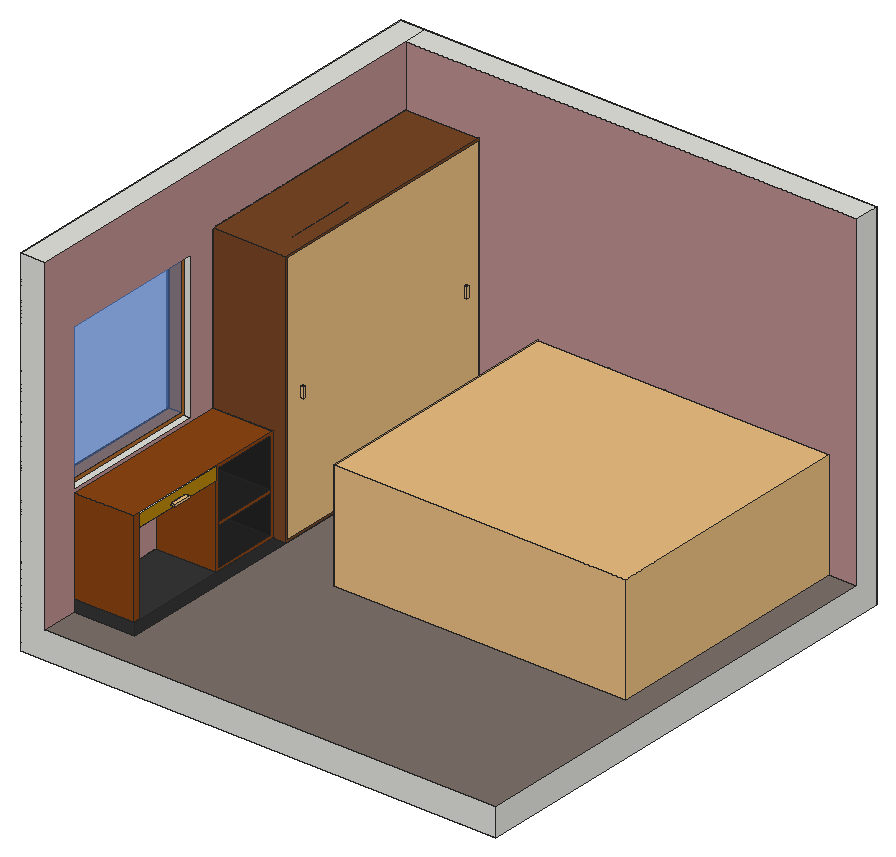
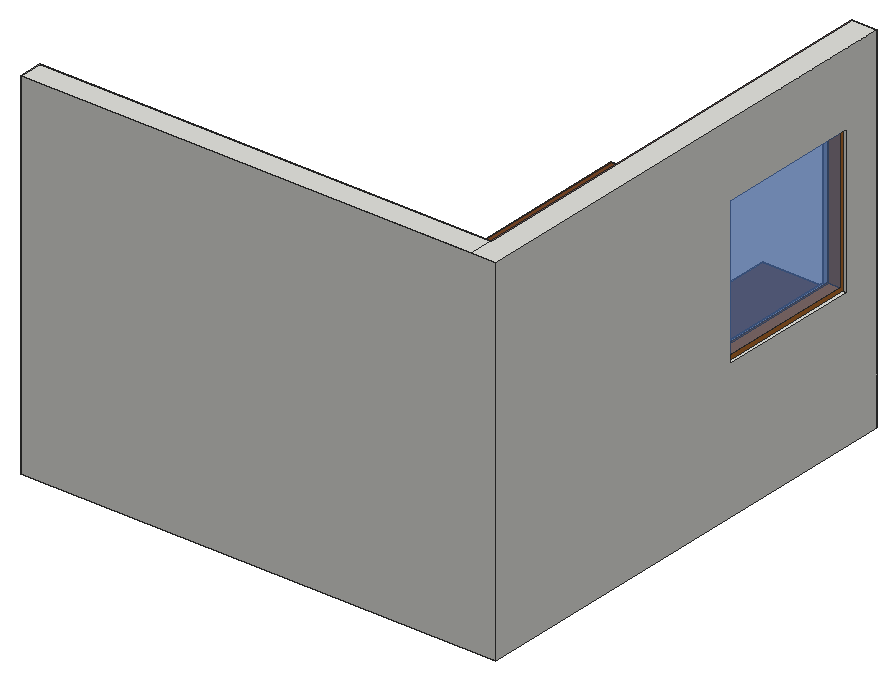
# SketchUp Ruby script. Lengths in inches.
U = 1.inch
M = Sketchup.active_model
def pt(a) = Geom::Point3d.new(a.map { |v| v * U })
def face(e, loops, mat)
  f = e.add_face(loops[0].map { |a| pt(a) })
  loops[1..].each { |l| e.add_face(l.map { |a| pt(a) }).erase! }
  f.material = f.back_material = mat if mat
  f
end
# faces: each face lists its corners as indices into pts; further lists are holes
def faces(e, pts, list, mat = nil) = list.each { |f| face(e, (f[0].is_a?(Array) ? f : [f]).map { |l| l.map { |i| pts[i] } }, mat) }
# xy, xz, yz: faces in a plane at the given z, y or x. An outline is a flat list of corners, or four numbers for a rectangle; further outlines are holes
def ring(l) = l.size == 4 ? [[l[0], l[1]], [l[2], l[1]], [l[2], l[3]], [l[0], l[3]]] : l.each_slice(2).to_a
def flat(e, list, mat, &to3) = list.each { |f| face(e, (f[0].is_a?(Array) ? f : [f]).map { |l| ring(l).map { |u, v| to3.(u, v) } }, mat) }
def xy(e, z, list, mat = nil) = flat(e, list, mat) { |x, y| [x, y, z] }
def xz(e, y, list, mat = nil) = flat(e, list, mat) { |x, z| [x, y, z] }
def yz(e, x, list, mat = nil) = flat(e, list, mat) { |y, z| [x, y, z] }
def lines(e, pts, list) = list.each { |a, b| e.add_line(pt(pts[a]), pt(pts[b])) }
# prism: a flat outline (further loops are holes) pulled along v
def prism(e, loops, v, mat = nil)
  f = face(e, loops, mat); d = Geom::Vector3d.new(v.map { |x| x * U })
  f.pushpull(f.normal.samedirection?(d) ? d.length : -d.length)
end
def box(e, o, s, mat = nil) = prism(e, [[o, [o[0] + s[0], o[1], o[2]], [o[0] + s[0], o[1] + s[1], o[2]], [o[0], o[1] + s[1], o[2]]]], [0, 0, s[2]], mat)
def at(x, y, z, deg = 0) = Geom::Transformation.translation(pt([x, y, z])) * Geom::Transformation.rotation(ORIGIN, Z_AXIS, deg.degrees)
def axes(o, x, y, z) = Geom::Transformation.new([*x, 0, *y, 0, *z, 0, *pt(o).to_a, 1])
def part(name) = M.definitions.add(name)
# library, detail: a bought-in or finely detailed component or shape, given as its bounding box
def library(name, o, s) = part(name).tap { |d| box(d.entities, o, s) }
def detail(e, o, s) = box(e.add_group.entities, o, s)
def put(e, d, t, mat = nil) = e.add_instance(d, t).tap { |i| i.material = mat if mat }
def group(e, t, mat = nil) = e.add_group.tap { |g| g.transformation = t; g.material = mat if mat }.entities
root = M.entities
M.materials.add("[0043_SaddleBrown]").color = [139, 69, 19]
M.materials.add("[0044_DarkGoldenrod]").color = [184, 134, 11]
M.materials.add("[0119_RosyBrown]").color = [188, 143, 143]
M.materials.add("[0136_Charcoal]").color = [35, 35, 35]
M.materials.add("[Color E01]").color = [255, 255, 204]
M.materials.add("[Color M00]").color = [255, 255, 255]
M.materials.add("[Slate Light Tile]").color = [54, 54, 54]
M.materials.add("[Tile Checker BW]").color = [125, 112, 107]
M.materials.add("[Translucent_Glass_Blue]").color = [100, 149, 237]
M.materials["[Translucent_Glass_Blue]"].alpha = 0.5
M.materials.add("[Wood Veneer 01]").color = [120, 70, 37]
M.materials.add("[Wood_Bamboo_Medium]").color = [177, 105, 43]
c1 = library("Platform bed",[0,0,0],[83.59,95.6,35.43])
c2 = part("Untitled")
xy(c2.entities,34.68,[[46.57,0,194.75,6.75]])
xy(c2.entities,36.94,[[49.13,0,192.19,6.75]],"[Wood_Bamboo_Medium]")
xy(c2.entities,126.69,[[49.13,0,192.19,6.75]],"[Wood_Bamboo_Medium]")
xy(c2.entities,128.49,[[46.57,0,194.75,6.75]],"[Wood_Bamboo_Medium]")
xz(c2.entities,0,[[49.13,36.94,192.19,126.69]],"[Translucent_Glass_Blue]")
xz(c2.entities,0,[[[46.57,34.68,194.75,128.49],[49.13,36.94,192.19,126.69]]],"[Wood_Bamboo_Medium]")
xz(c2.entities,6.75,[[49.13,36.94,192.19,126.69]],"[Translucent_Glass_Blue]")
xz(c2.entities,6.75,[[[46.57,34.68,194.75,128.49],[49.13,36.94,192.19,126.69]]],"[Wood_Bamboo_Medium]")
yz(c2.entities,46.57,[[0,34.68,6.75,128.49]],"[Wood_Bamboo_Medium]")
yz(c2.entities,49.13,[[0,36.94,6.75,126.69]],"[Wood_Bamboo_Medium]")
yz(c2.entities,192.19,[[0,36.94,6.75,126.69]],"[Wood_Bamboo_Medium]")
yz(c2.entities,194.75,[[0,34.68,6.75,128.49]])
c3 = library("1-POIGNEE CLC2\#1",[-3.03,-0.375,0],[6.06,0.75,1.42])
c4 = library("Group\#2",[128,-0.28,0],[77.78,1.7,82.58])
put(root,c1,at(146.95,64.41,9,90))
put(root,c2,axes([5.625,-3.08,27.26],[0,0.32391,0],[-0.62,0,0],[0,0,0.51166]))
g1 = group(root,at(0,0,0))
xy(g1,0,[[0,0,156,156]])
xy(g1,9,[[8,0,156,148]],"[Tile Checker BW]")
xy(g1,45,[[0,12,8,60]])
xy(g1,93,[[0,12,8,60]])
xy(g1,117,[[0,0,8,156],[8,148,156,156]])
xz(g1,0,[[0,0,156,0,156,9,8,9,8,117,0,117]])
xz(g1,12,[[0,45,8,93]])
xz(g1,60,[[0,45,8,93]])
xz(g1,148,[[8,9,156,117]],"[0119_RosyBrown]")
xz(g1,156,[[0,0,156,117]])
yz(g1,0,[[[0,0,156,117],[12,45,60,93]]])
yz(g1,8,[[[0,9,148,117],[12,45,60,93]]],"[0119_RosyBrown]")
yz(g1,156,[[0,0,156,0,156,117,148,117,148,9,0,9]])
g2 = group(root,at(8,68.01,9))
detail(g2,[24,6.31,44.22],[1.42,0.75,3.58])
detail(g2,[24,73.44,44.22],[1.42,0.75,3.58])
g3 = group(g2,at(24,0.79,0,90))
xy(g3,0,[[-56.8,4,79.2,24]])
xy(g3,4,[[0,4,79.2,24]])
xy(g3,4,[[-56.8,4,-54.8,4.25],[-23.37,4,0,4.25]],"[Color M00]")
xy(g3,4,[[-54.8,4,-23.37,24],[-56.8,4.25,-54.8,24],[-23.37,4.25,0,24]],"[Slate Light Tile]")
xy(g3,4,[[0,0,79.2,4]],"[Wood Veneer 01]")
xy(g3,4.71,[[0.71,0,78.49,0.71],[0.71,0.71,78.49,1.42],[0.71,1.42,39.25,22],[39.95,1.42,78.49,22]])
xy(g3,4.71,[[-22.66,4.25,-0.71,24]],"[0136_Charcoal]")
xy(g3,17.47,[[-22.66,4.25,-0.71,24]],"[0136_Charcoal]")
xy(g3,18.18,[[-22.66,4.25,-0.71,24]],"[0136_Charcoal]")
xy(g3,21.65,[[0.71,1.42,19.62,22],[19.62,1.42,20.33,22],[20.33,1.42,39.25,22],[39.95,1.42,58.87,22],[58.87,1.42,59.58,22],
  [59.58,1.42,78.49,22]])
xy(g3,22.35,[[0.71,1.42,19.62,22],[20.33,1.42,39.25,22],[39.95,1.42,58.87,22],[59.58,1.42,78.49,22]])
xy(g3,30.95,[[-54.8,4.25,-23.37,24]],"[Color M00]")
xy(g3,31.11,[[-54.64,4,-23.52,4.25]],"[Color M00]")
xy(g3,34.49,[[-22.66,4.25,-0.71,24]],"[0136_Charcoal]")
xy(g3,35.04,[[-54.64,4,-23.52,4.25]],"[Color M00]")
xy(g3,35.2,[[-56.8,4.25,0,24]],"[0043_SaddleBrown]")
xy(g3,40,[[0.71,1.42,19.62,22],[20.33,1.42,39.25,22],[39.95,1.42,58.87,22],[59.58,1.42,78.49,22]])
xy(g3,46,[[0.71,1.42,39.25,22],[39.95,1.42,78.49,22]])
xy(g3,59.41,[[39.95,1.42,58.87,22],[58.87,1.42,59.58,22],[59.58,1.42,78.49,22]])
xy(g3,60.12,[[39.95,1.42,58.87,22],[59.58,1.42,78.49,22]])
xy(g3,73.17,[[39.95,1.42,58.87,22],[59.58,1.42,78.49,22]])
xy(g3,73.88,[[39.95,1.42,59.22,22],[59.22,1.42,78.49,22]])
xy(g3,82.29,[[0.71,11.65,39.25,11.71],[0.71,11.71,39.25,11.77]])
xy(g3,84.29,[[0.71,11.65,39.25,11.71],[0.71,11.71,39.25,11.77]])
xy(g3,87.29,[[0.71,0,78.49,0.71],[0.71,0.71,78.49,1.42],[0.71,1.42,39.25,22],[39.95,1.42,78.49,22]])
xy(g3,88,[[0,0,79.2,24]],"[Wood Veneer 01]")
xz(g3,0,[[[0,4,79.2,88],[0.71,4.71,78.49,87.29]]],"[Wood Veneer 01]")
xz(g3,1.42,[[39.25,4.71,39.95,87.29],[0.71,21.65,39.25,21.65,39.25,22.35,20.33,22.35,20.33,40,19.62,40,19.62,22.35,0.71,22.35],[39.95,21.65,78.49,21.65,78.49,22.35,59.58,22.35,59.58,40,58.87,40,58.87,22.35,39.95,22.35],[[0.71,40,39.25,46],[0.83,40.12,19.86,45.88],[20.1,40.12,39.13,45.88]],[[39.95,40,78.49,46],[59.34,40.12,78.375,45.88],[40.07,40.12,59.1,45.88]],
  [0.83,40.12,19.86,45.88],[20.1,40.12,39.13,45.88],[40.07,40.12,59.1,45.88],[59.34,40.12,78.375,45.88],[39.95,59.41,78.49,60.12],
  [58.87,60.12,59.58,73.17],[39.95,73.17,78.49,73.88]])
xz(g3,4,[[-54.64,31.11,-23.52,35.04]],"[0044_DarkGoldenrod]")
xz(g3,4,[[-56.8,0,79.2,4]],"[Slate Light Tile]")
xz(g3,4.25,[[-56.8,4,-54.8,35.2],[[-23.37,4,0,35.2],[-22.66,4.71,-0.71,34.49]],[-22.66,17.47,-0.71,18.18]],"[0043_SaddleBrown]")
xz(g3,4.25,[[[-54.8,30.95,-23.37,35.2],[-54.64,31.11,-23.52,35.04]]],"[Color M00]")
xz(g3,10.71,[[0.71,83.23,39.25,83.29],[0.71,83.29,39.25,83.35]])
xz(g3,12.71,[[0.71,83.23,39.25,83.29],[0.71,83.29,39.25,83.35]])
xz(g3,22,[[0.71,4.71,39.25,21.65],[39.95,4.71,78.49,21.65],[0.71,22.35,19.62,40],[20.33,22.35,39.25,40],[39.95,22.35,58.87,40],
  [59.58,22.35,78.49,40],[0.71,46,39.25,87.29],[39.95,46,78.49,59.41],[39.95,60.12,58.87,73.17],[59.58,60.12,78.49,73.17],
  [39.95,73.88,78.49,87.29]])
xz(g3,24,[[-56.8,0,79.2,4],[0,4,79.2,88]])
xz(g3,24,[[[-56.8,4,-56.8,35.2,0,35.2,0,4,-23.37,4,-23.37,30.95,-54.8,30.95,-54.8,4],[-22.66,18.18,-0.71,34.49],[-22.66,4.71,-0.71,17.47]]],"[Slate Light Tile]")
yz(g3,-56.8,[[4.25,4,24,35.2]],"[0043_SaddleBrown]")
yz(g3,-56.8,[[4,0,24,4]],"[Slate Light Tile]")
yz(g3,-54.8,[[4.25,4,24,30.95]],"[0043_SaddleBrown]")
yz(g3,-54.64,[[4,31.11,4.25,35.04]],"[Color M00]")
yz(g3,-23.52,[[4,31.11,4.25,35.04]],"[Color M00]")
yz(g3,-23.37,[[4.25,4,24,30.95]],"[0043_SaddleBrown]")
yz(g3,-22.66,[[4.25,4.71,24,17.47],[4.25,18.18,24,30.95],[4.25,30.95,24,34.49]],"[0136_Charcoal]")
yz(g3,-0.71,[[4.25,4.71,24,17.47],[4.25,18.18,24,34.49]],"[0136_Charcoal]")
yz(g3,0,[[4.25,4,24,35.2]],"[Slate Light Tile]")
yz(g3,0,[[0,4,0,88,24,88,24,35.2,4.25,35.2,4.25,4]],"[Wood Veneer 01]")
yz(g3,0.71,[[0,4.71,0.71,87.29],[0.71,4.71,1.42,87.29],[1.42,4.71,22,21.65],[1.42,22.35,22,40],[[1.42,46,22,87.29],[11.65,82.29,11.58,82.3,11.46,82.32,11.34,82.36,11.28,82.39,11.23,82.42,11.17,82.45,11.12,82.48,11.07,82.52,11.02,82.5625,10.98,82.61,10.9375,82.65,10.9,82.7,10.86,82.76,10.83,82.81,10.8,82.87,10.78,82.92,10.74,83.04,10.73,83.1,10.72,83.17,10.71,83.23,10.71,83.35,10.72,83.42,10.74,83.54,10.8,83.72,10.83,83.77,10.86,83.83,10.9,83.88,10.9375,83.93,10.98,83.98,11.02,84.02,11.07,84.0625,11.12,84.1,11.17,84.14,11.23,84.17,11.28,84.2,11.46,84.26,11.58,84.28,11.65,84.29,11.77,84.29,11.83,84.28,11.9,84.27,11.96,84.26,12.08,84.22,12.13,84.2,12.19,84.17,12.24,84.14,12.3,84.1,12.35,84.0625,12.39,84.02,12.4375,83.98,12.48,83.93,12.52,83.88,12.55,83.83,12.58,83.77,12.61,83.72,12.64,83.66,12.68,83.54,12.7,83.42,12.71,83.35,12.71,83.23,12.7,83.17,12.69,83.1,12.68,83.04,12.64,82.92,12.61,82.87,12.58,82.81,12.55,82.76,12.52,82.7,12.48,82.65,12.4375,82.61,12.39,82.5625,12.35,82.52,12.3,82.48,12.24,82.45,12.19,82.42,12.13,82.39,12.08,82.36,11.96,82.32,11.9,82.31,11.83,82.3,11.77,82.29]]])
yz(g3,19.62,[[1.42,22.35,22,40]])
yz(g3,20.33,[[1.42,22.35,22,40]])
yz(g3,39.25,[[1.42,4.71,22,21.65],[1.42,22.35,22,40],[[1.42,46,22,87.29],[11.65,82.29,11.77,82.29,11.83,82.3,11.9,82.31,11.96,82.32,12.08,82.36,12.13,82.39,12.19,82.42,12.24,82.45,12.3,82.48,12.35,82.52,12.39,82.5625,12.4375,82.61,12.48,82.65,12.52,82.7,12.55,82.76,12.58,82.81,12.61,82.87,12.64,82.92,12.68,83.04,12.69,83.1,12.7,83.17,12.71,83.23,12.71,83.35,12.7,83.42,12.68,83.54,12.64,83.66,12.61,83.72,12.58,83.77,12.55,83.83,12.52,83.88,12.48,83.93,12.4375,83.98,12.39,84.02,12.35,84.0625,12.3,84.1,12.24,84.14,12.19,84.17,12.13,84.2,12.08,84.22,11.96,84.26,11.9,84.27,11.83,84.28,11.77,84.29,11.65,84.29,11.58,84.28,11.46,84.26,11.28,84.2,11.23,84.17,11.17,84.14,11.12,84.1,11.07,84.0625,11.02,84.02,10.98,83.98,10.9375,83.93,10.9,83.88,10.86,83.83,10.83,83.77,10.8,83.72,10.74,83.54,10.72,83.42,10.71,83.35,10.71,83.23,10.72,83.17,10.73,83.1,10.74,83.04,10.78,82.92,10.8,82.87,10.83,82.81,10.86,82.76,10.9,82.7,10.9375,82.65,10.98,82.61,11.02,82.5625,11.07,82.52,11.12,82.48,11.17,82.45,11.23,82.42,11.28,82.39,11.34,82.36,11.46,82.32,11.58,82.3]]])
yz(g3,39.95,[[1.42,4.71,22,21.65],[1.42,22.35,22,40],[1.42,46,22,59.41],[1.42,60.12,22,73.17],[1.42,73.88,22,87.29]])
yz(g3,58.87,[[1.42,22.35,22,40],[1.42,60.12,22,73.17]])
yz(g3,59.58,[[1.42,22.35,22,40],[1.42,60.12,22,73.17]])
yz(g3,78.49,[[0,4.71,0.71,87.29],[0.71,4.71,1.42,87.29],[1.42,4.71,22,21.65],[1.42,22.35,22,40],[1.42,46,22,59.41],
  [1.42,60.12,22,73.17],[1.42,73.88,22,87.29]])
yz(g3,79.2,[[4,0,24,4]],"[Slate Light Tile]")
yz(g3,79.2,[[0,4,24,88]],"[Wood Veneer 01]")
p = [[0.71,11.34,82.36],[0.71,11.4,82.34],[39.25,11.4,82.34],[39.25,11.34,82.36],[0.71,11.46,82.32],[39.25,11.46,82.32],
  [0.71,11.52,82.31],[39.25,11.52,82.31],[0.71,11.58,82.3],[39.25,11.58,82.3],[0.71,11.65,82.29],[39.25,11.65,82.29],
  [0.71,11.77,82.29],[0.71,11.83,82.3],[39.25,11.83,82.3],[39.25,11.77,82.29],[0.71,11.9,82.31],[39.25,11.9,82.31],
  [0.71,11.96,82.32],[39.25,11.96,82.32],[0.71,12.02,82.34],[39.25,12.02,82.34],[0.71,12.08,82.36],[39.25,12.08,82.36],
  [0.71,11.12,82.48],[0.71,11.17,82.45],[39.25,11.17,82.45],[39.25,11.12,82.48],[0.71,11.23,82.42],[39.25,11.23,82.42],
  [0.71,11.28,82.39],[39.25,11.28,82.39],[0.71,12.13,82.39],[39.25,12.13,82.39],[0.71,12.19,82.42],[39.25,12.19,82.42],
  [0.71,12.24,82.45],[39.25,12.24,82.45],[0.71,12.3,82.48],[39.25,12.3,82.48],[0.71,11.02,82.5625],[0.71,11.07,82.52],
  [39.25,11.07,82.52],[39.25,11.02,82.5625],[0.71,12.35,82.52],[39.25,12.35,82.52],[0.71,12.39,82.5625],[39.25,12.39,82.5625],
  [0.71,10.9375,82.65],[0.71,10.98,82.61],[39.25,10.98,82.61],[39.25,10.9375,82.65],[0.71,12.4375,82.61],[39.25,12.4375,82.61],
  [0.71,12.48,82.65],[39.25,12.48,82.65],[0.71,10.86,82.76],[0.71,10.9,82.7],[39.25,10.9,82.7],[39.25,10.86,82.76],
  [0.71,12.52,82.7],[39.25,12.52,82.7],[0.71,12.55,82.76],[39.25,12.55,82.76],[0.71,10.8,82.87],[0.71,10.83,82.81],
  [39.25,10.83,82.81],[39.25,10.8,82.87],[0.71,12.58,82.81],[39.25,12.58,82.81],[0.71,12.61,82.87],[39.25,12.61,82.87],
  [0.71,10.76,82.98],[0.71,10.78,82.92],[39.25,10.78,82.92],[39.25,10.76,82.98],[0.71,12.64,82.92],[39.25,12.64,82.92],
  [0.71,12.66,82.98],[39.25,12.66,82.98],[0.71,10.73,83.1],[0.71,10.74,83.04],[39.25,10.74,83.04],[39.25,10.73,83.1],
  [0.71,12.68,83.04],[39.25,12.68,83.04],[0.71,12.69,83.1],[39.25,12.69,83.1],[0.71,10.72,83.17],[39.25,10.72,83.17],
  [0.71,12.7,83.17],[39.25,12.7,83.17],[0.71,10.71,83.23],[39.25,10.71,83.23],[0.71,12.71,83.23],[39.25,12.71,83.23],
  [0.71,10.73,83.48],[0.71,10.72,83.42],[39.25,10.72,83.42],[39.25,10.73,83.48],[0.71,10.71,83.35],[39.25,10.71,83.35],
  [0.71,12.71,83.35],[0.71,12.7,83.42],[39.25,12.7,83.42],[39.25,12.71,83.35],[0.71,12.69,83.48],[39.25,12.69,83.48],
  [0.71,10.76,83.6],[0.71,10.74,83.54],[39.25,10.74,83.54],[39.25,10.76,83.6],[0.71,12.68,83.54],[39.25,12.68,83.54],
  [0.71,12.66,83.6],[39.25,12.66,83.6],[0.71,10.78,83.66],[39.25,10.78,83.66],[0.71,12.64,83.66],[39.25,12.64,83.66],
  [0.71,10.83,83.77],[0.71,10.8,83.72],[39.25,10.8,83.72],[39.25,10.83,83.77],[0.71,12.61,83.72],[39.25,12.61,83.72],
  [0.71,12.58,83.77],[39.25,12.58,83.77],[0.71,10.86,83.83],[39.25,10.86,83.83],[0.71,10.9,83.88],[39.25,10.9,83.88],
  [0.71,12.55,83.83],[0.71,12.52,83.88],[39.25,12.52,83.88],[39.25,12.55,83.83],[0.71,10.98,83.98],[0.71,10.9375,83.93],
  [39.25,10.9375,83.93],[39.25,10.98,83.98],[0.71,12.48,83.93],[0.71,12.4375,83.98],[39.25,12.4375,83.98],[39.25,12.48,83.93],
  [0.71,11.07,84.0625],[0.71,11.02,84.02],[39.25,11.02,84.02],[39.25,11.07,84.0625],[0.71,12.39,84.02],[0.71,12.35,84.0625],
  [39.25,12.35,84.0625],[39.25,12.39,84.02],[0.71,11.17,84.14],[0.71,11.12,84.1],[39.25,11.12,84.1],[39.25,11.17,84.14],
  [0.71,11.23,84.17],[39.25,11.23,84.17],[0.71,12.3,84.1],[0.71,12.24,84.14],[39.25,12.24,84.14],[39.25,12.3,84.1],
  [0.71,12.19,84.17],[39.25,12.19,84.17],[0.71,11.28,84.2],[39.25,11.28,84.2],[0.71,11.4,84.24],[0.71,11.34,84.22],
  [39.25,11.34,84.22],[39.25,11.4,84.24],[0.71,11.46,84.26],[39.25,11.46,84.26],[0.71,12.08,84.22],[0.71,12.02,84.24],
  [39.25,12.02,84.24],[39.25,12.08,84.22],[0.71,11.96,84.26],[39.25,11.96,84.26],[0.71,12.13,84.2],[39.25,12.13,84.2],
  [0.71,11.58,84.28],[0.71,11.52,84.27],[39.25,11.52,84.27],[39.25,11.58,84.28],[0.71,11.65,84.29],[39.25,11.65,84.29],
  [0.71,11.9,84.27],[0.71,11.83,84.28],[39.25,11.83,84.28],[39.25,11.9,84.27],[0.71,11.77,84.29],[39.25,11.77,84.29],
  [-0.79,22,22.35],[0.71,22,22.35]]
faces(g3,p,[[0,1,2,3],[1,4,5,2],[4,6,7,5],[6,8,9,7],[8,10,11,9],[12,13,14,15],[13,16,17,14],[16,18,19,17],
  [18,20,21,19],[20,22,23,21],[24,25,26,27],[25,28,29,26],[28,30,31,29],[30,0,3,31],[22,32,33,23],[32,34,35,33],
  [34,36,37,35],[36,38,39,37],[40,41,42,43],[41,24,27,42],[38,44,45,39],[44,46,47,45],[48,49,50,51],[49,40,43,50],
  [46,52,53,47],[52,54,55,53],[56,57,58,59],[57,48,51,58],[54,60,61,55],[60,62,63,61],[64,65,66,67],[65,56,59,66],
  [62,68,69,63],[68,70,71,69],[72,73,74,75],[73,64,67,74],[70,76,77,71],[76,78,79,77],[80,81,82,83],[81,72,75,82],
  [78,84,85,79],[84,86,87,85],[88,80,83,89],[86,90,91,87],[92,88,89,93],[90,94,95,91],[96,97,98,99],[97,100,101,98],
  [102,103,104,105],[103,106,107,104],[108,109,110,111],[109,96,99,110],[106,112,113,107],[112,114,115,113],[116,108,111,117],[114,118,119,115],
  [120,121,122,123],[121,116,117,122],[118,124,125,119],[124,126,127,125],[128,120,123,129],[130,128,129,131],[132,133,134,135],[126,132,135,127],
  [136,137,138,139],[137,130,131,138],[140,141,142,143],[133,140,143,134],[144,145,146,147],[145,136,139,146],[148,149,150,151],[141,148,151,142],
  [152,153,154,155],[153,144,147,154],[156,152,155,157],[158,159,160,161],[159,162,163,160],[149,158,161,150],[164,156,157,165],[166,167,168,169],
  [167,164,165,168],[170,166,169,171],[172,173,174,175],[173,176,177,174],[162,178,179,163],[178,172,175,179],[180,181,182,183],[181,170,171,182],
  [184,180,183,185],[186,187,188,189],[187,190,191,188],[176,186,189,177]])
lines(g3,p,[[192,193]])
put(g3,c3,axes([-39.08,4,32.36],[1,0,0],[0,0,1],[0,-1,0]))
put(g3,c4,at(-127.29,0,4.71),"[Color E01]")
